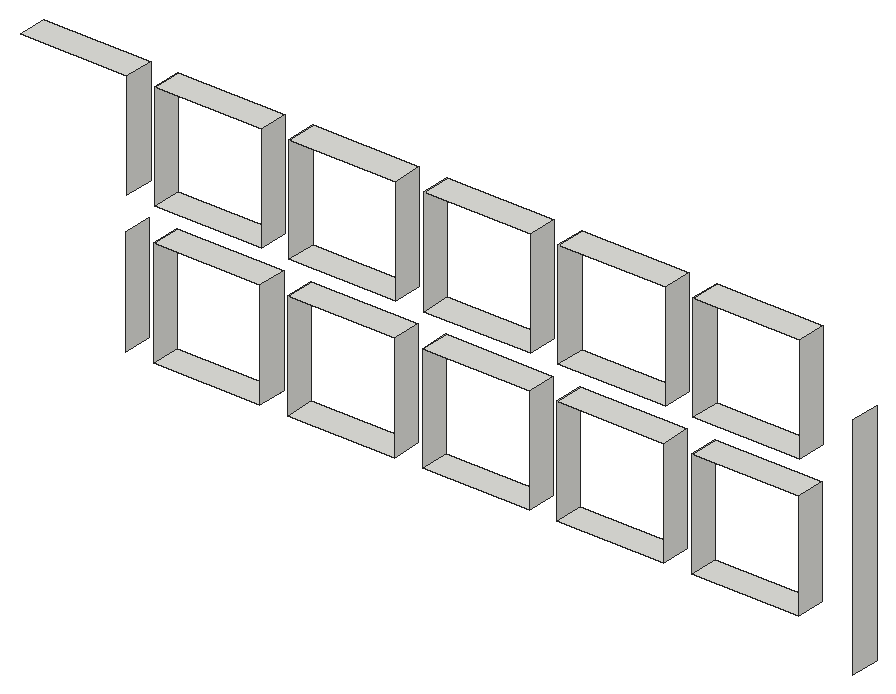
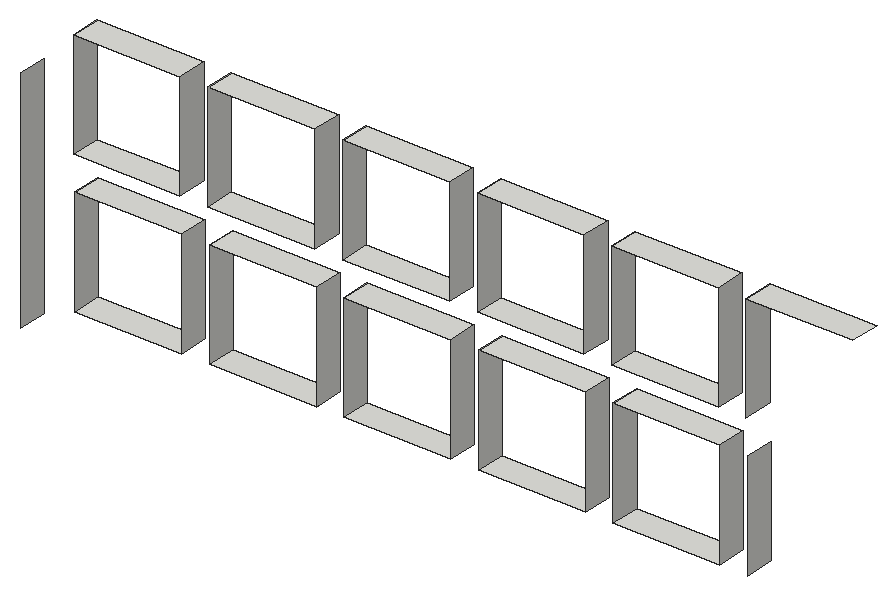
# SketchUp Ruby script. Lengths in inches.
U = 1.inch
M = Sketchup.active_model
def pt(a) = Geom::Point3d.new(a.map { |v| v * U })
def face(e, loops, mat)
  f = e.add_face(loops[0].map { |a| pt(a) })
  loops[1..].each { |l| e.add_face(l.map { |a| pt(a) }).erase! }
  f.material = f.back_material = mat if mat
  f
end
# faces: each face lists its corners as indices into pts; further lists are holes
def faces(e, pts, list, mat = nil) = list.each { |f| face(e, (f[0].is_a?(Array) ? f : [f]).map { |l| l.map { |i| pts[i] } }, mat) }
# xy, xz, yz: faces in a plane at the given z, y or x. An outline is a flat list of corners, or four numbers for a rectangle; further outlines are holes
def ring(l) = l.size == 4 ? [[l[0], l[1]], [l[2], l[1]], [l[2], l[3]], [l[0], l[3]]] : l.each_slice(2).to_a
def flat(e, list, mat, &to3) = list.each { |f| face(e, (f[0].is_a?(Array) ? f : [f]).map { |l| ring(l).map { |u, v| to3.(u, v) } }, mat) }
def xy(e, z, list, mat = nil) = flat(e, list, mat) { |x, y| [x, y, z] }
def xz(e, y, list, mat = nil) = flat(e, list, mat) { |x, z| [x, y, z] }
def yz(e, x, list, mat = nil) = flat(e, list, mat) { |y, z| [x, y, z] }
def lines(e, pts, list) = list.each { |a, b| e.add_line(pt(pts[a]), pt(pts[b])) }
# prism: a flat outline (further loops are holes) pulled along v
def prism(e, loops, v, mat = nil)
  f = face(e, loops, mat); d = Geom::Vector3d.new(v.map { |x| x * U })
  f.pushpull(f.normal.samedirection?(d) ? d.length : -d.length)
end
def box(e, o, s, mat = nil) = prism(e, [[o, [o[0] + s[0], o[1], o[2]], [o[0] + s[0], o[1] + s[1], o[2]], [o[0], o[1] + s[1], o[2]]]], [0, 0, s[2]], mat)
def at(x, y, z, deg = 0) = Geom::Transformation.translation(pt([x, y, z])) * Geom::Transformation.rotation(ORIGIN, Z_AXIS, deg.degrees)
def axes(o, x, y, z) = Geom::Transformation.new([*x, 0, *y, 0, *z, 0, *pt(o).to_a, 1])
def part(name) = M.definitions.add(name)
# library, detail: a bought-in or finely detailed component or shape, given as its bounding box
def library(name, o, s) = part(name).tap { |d| box(d.entities, o, s) }
def detail(e, o, s) = box(e.add_group.entities, o, s)
def put(e, d, t, mat = nil) = e.add_instance(d, t).tap { |i| i.material = mat if mat }
def group(e, t, mat = nil) = e.add_group.tap { |g| g.transformation = t; g.material = mat if mat }.entities
root = M.entities
xy(root,259.68,[[2258.08,480.14,2260.39,480.77],[2260.99,480.14,2263.3,480.77],[2263.9,480.14,2266.22,480.77],[2266.81,480.14,2269.13,480.77],[2269.73,480.14,2272.04,480.77]])
xy(root,262,[[2258.08,480.14,2260.39,480.77],[2260.99,480.14,2263.3,480.77],[2263.9,480.14,2266.22,480.77],[2266.81,480.14,2269.13,480.77],[2269.73,480.14,2272.04,480.77]])
xy(root,262.73,[[2258.11,480.14,2260.42,480.77],[2261.02,480.14,2263.33,480.77],[2263.93,480.14,2266.24,480.77],[2266.84,480.14,2269.16,480.77],[2269.76,480.14,2272.07,480.77]])
xy(root,265.04,[[2255.2,480.14,2257.51,480.77],[2258.11,480.14,2260.42,480.77],[2261.02,480.14,2263.33,480.77],[2263.93,480.14,2266.24,480.77],[2266.84,480.14,2269.16,480.77],
  [2269.76,480.14,2272.07,480.77]])
yz(root,2257.48,[[480.14,259.68,480.77,262]])
yz(root,2257.51,[[480.14,262.73,480.77,265.04]])
yz(root,2258.08,[[480.14,259.68,480.77,262]])
yz(root,2258.11,[[480.14,262.73,480.77,265.04]])
yz(root,2260.39,[[480.14,259.68,480.77,262]])
yz(root,2260.42,[[480.14,262.73,480.77,265.04]])
yz(root,2260.99,[[480.14,259.68,480.77,262]])
yz(root,2261.02,[[480.14,262.73,480.77,265.04]])
yz(root,2263.3,[[480.14,259.68,480.77,262]])
yz(root,2263.33,[[480.14,262.73,480.77,265.04]])
yz(root,2263.9,[[480.14,259.68,480.77,262]])
yz(root,2263.93,[[480.14,262.73,480.77,265.04]])
yz(root,2266.22,[[480.14,259.68,480.77,262]])
yz(root,2266.24,[[480.14,262.73,480.77,265.04]])
yz(root,2266.81,[[480.14,259.68,480.77,262]])
yz(root,2266.84,[[480.14,262.73,480.77,265.04]])
yz(root,2269.13,[[480.14,259.68,480.77,262]])
yz(root,2269.16,[[480.14,262.73,480.77,265.04]])
yz(root,2269.73,[[480.14,259.68,480.77,262]])
yz(root,2269.76,[[480.14,262.73,480.77,265.04]])
yz(root,2272.04,[[480.14,259.68,480.77,262]])
yz(root,2272.07,[[480.14,262.73,480.77,265.04]])
yz(root,2273.22,[[480.14,258.95,480.77,263.89]])
